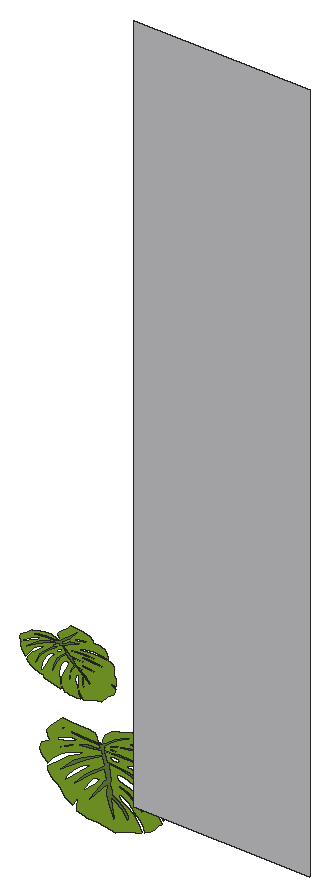
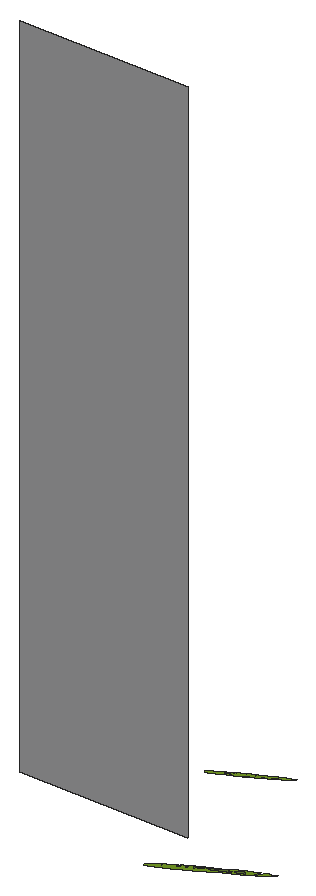
# SketchUp Ruby script. Lengths in inches.
U = 1.inch
M = Sketchup.active_model
def pt(a) = Geom::Point3d.new(a.map { |v| v * U })
def face(e, loops, mat)
  f = e.add_face(loops[0].map { |a| pt(a) })
  loops[1..].each { |l| e.add_face(l.map { |a| pt(a) }).erase! }
  f.material = f.back_material = mat if mat
  f
end
# faces: each face lists its corners as indices into pts; further lists are holes
def faces(e, pts, list, mat = nil) = list.each { |f| face(e, (f[0].is_a?(Array) ? f : [f]).map { |l| l.map { |i| pts[i] } }, mat) }
# xy, xz, yz: faces in a plane at the given z, y or x. An outline is a flat list of corners, or four numbers for a rectangle; further outlines are holes
def ring(l) = l.size == 4 ? [[l[0], l[1]], [l[2], l[1]], [l[2], l[3]], [l[0], l[3]]] : l.each_slice(2).to_a
def flat(e, list, mat, &to3) = list.each { |f| face(e, (f[0].is_a?(Array) ? f : [f]).map { |l| ring(l).map { |u, v| to3.(u, v) } }, mat) }
def xy(e, z, list, mat = nil) = flat(e, list, mat) { |x, y| [x, y, z] }
def xz(e, y, list, mat = nil) = flat(e, list, mat) { |x, z| [x, y, z] }
def yz(e, x, list, mat = nil) = flat(e, list, mat) { |y, z| [x, y, z] }
def lines(e, pts, list) = list.each { |a, b| e.add_line(pt(pts[a]), pt(pts[b])) }
# prism: a flat outline (further loops are holes) pulled along v
def prism(e, loops, v, mat = nil)
  f = face(e, loops, mat); d = Geom::Vector3d.new(v.map { |x| x * U })
  f.pushpull(f.normal.samedirection?(d) ? d.length : -d.length)
end
def box(e, o, s, mat = nil) = prism(e, [[o, [o[0] + s[0], o[1], o[2]], [o[0] + s[0], o[1] + s[1], o[2]], [o[0], o[1] + s[1], o[2]]]], [0, 0, s[2]], mat)
def at(x, y, z, deg = 0) = Geom::Transformation.translation(pt([x, y, z])) * Geom::Transformation.rotation(ORIGIN, Z_AXIS, deg.degrees)
def axes(o, x, y, z) = Geom::Transformation.new([*x, 0, *y, 0, *z, 0, *pt(o).to_a, 1])
def part(name) = M.definitions.add(name)
# library, detail: a bought-in or finely detailed component or shape, given as its bounding box
def library(name, o, s) = part(name).tap { |d| box(d.entities, o, s) }
def detail(e, o, s) = box(e.add_group.entities, o, s)
def put(e, d, t, mat = nil) = e.add_instance(d, t).tap { |i| i.material = mat if mat }
def group(e, t, mat = nil) = e.add_group.tap { |g| g.transformation = t; g.material = mat if mat }.entities
root = M.entities
M.materials.add("[0059_DarkOliveGreen]").color = [85, 107, 47]
M.materials.add("[0061_OliveDrab]").color = [107, 142, 35]
M.materials.add("[Polished Concrete New]").color = [200, 200, 203]
xz(root,148.8,[[547.38,7.8125,584.28,155.375]],"[Polished Concrete New]")
p = [[526.03,158.54,12.29],[524.84,158.39,12.53],[524.12,156.41,11.83],[524.16,155.22,11.28],[524.77,154.53,10.82],[525.48,154.2,10.48],
  [524.78,153.11,10.18],[525.2,152.12,9.62],[525.96,151.55,9.17],[527.39,151.0625,8.58],[527.87,150.84,8.36],[527.96,152.03,8.87],
  [528.62,153.25,9.25],[529.63,154.43,9.52],[530.89,155.28,9.58],[531.28,155.4375,9.55],[531.42,155.37,9.48],[531.26,155.08,9.39],
  [529.98,153.69,9.1],[529.14,152.47,8.77],[528.45,151.15,8.35],[528.24,150.44,8.09],[528.55,149.84,7.74],[529.26,149.51,7.41],
  [530.45,149.15,6.94],[531.53,148.86,6.53],[532.09,148.71,6.32],[533.02,148.16,5.83],[534.1,147.77,5.38],[535.19,147.54,5],
  [535.77,147.39,4.78],[535.6875,148.05,5.1],[535.58,149.06,5.58],[536.6875,147.26,4.49],[537,147.05,4.3125],[538.01,146.99,4.02],
  [539.03,146.92,3.73],[541.36,147.39,3.34],[544.66,147.61,2.59],[546,148.72,2.75],[547.33,149.5,2.75],[548.19,149.9375,2.73],
  [546.53,151.07,3.66],[545.23,151.69,4.28],[543.36,152.125,4.95],[542.05,152.39,5.41],[541.4,152.69,5.71],[540.88,152.94,5.96],
  [540.88,153.11,6.03],[541.24,153.17,5.97],[542.27,153.04,5.64],[543.15,152.82,5.32],[544.96,152.125,4.54],[546.48,151.5,3.87],
  [547.4375,151.15,3.46],[548.07,150.74,3.12],[548.54,150.3125,2.81],[549.22,150.98,2.93],[549.54,151.56,3.11],[549.71,152.07,3.29],
  [549.79,152.48,3.46],[549.96,152.96,3.625],[548.47,153.84,4.41],[547.06,154.3125,4.98],[545.82,154.53,5.4],[543.51,154.78,6.1],
  [541.76,154.85,6.59],[540.27,154.95,7.02],[539.16,155.1,7.37],[538.63,155.35,7.62],[538.6,155.6875,7.78],[539.43,155.83,7.625],
  [540.57,155.92,7.37],[542.57,155.75,6.78],[544.72,155.32,6.04],[547.1,154.65,5.125],[549.78,153.62,3.97],[550.08,155.34,4.67],
  [550.12,156.36,5.11],[549.7,156.81,5.42],[548.72,157.28,5.88],[547.51,157.55,6.32],[545.89,157.65,6.78],[544.51,157.73,7.17],
  [542.47,157.82,7.73],[540.96,157.76,8.1],[539.78,157.71,8.38],[539.21,157.64,8.5],[538.88,157.8,8.65],[539.23,158.04,8.67],
  [540.1,158.34,8.58],[541.47,158.49,8.29],[544.24,158.36,7.52],[545.87,158.17,7.02],[547.32,157.92,6.53],[547.99,157.67,6.25],
  [549.33,157.28,5.73],[549.38,157.5625,5.84],[549.05,158.55,6.37],[548.7,159.44,6.86],[547.35,160.44,7.66],[545.9375,160.625,8.1],
  [543.68,160.48,8.62],[541.69,160.07,8.94],[539.875,159.76,9.28],[539.08,159.61,9.41],[538.63,159.64,9.54],[538.68,159.8125,9.61],
  [539.6,160.1875,9.54],[541.83,160.71,9.2],[543.63,160.86,8.8],[546.51,160.86,8.06],[545.06,162.05,8.97],[543.6,162.67,9.62],
  [542.37,162.77,9.99],[541.74,162.57,10.06],[539.83,161.91,10.25],[538.42,161.31,10.35],[537.31,160.93,10.46],[536.86,160.88,10.55],
  [536.72,161.05,10.66],[536.96,161.21,10.68],[538.74,162.01,10.58],[540.17,162.47,10.41],[541.44,162.76,10.22],[542.41,162.97,10.0625],
  [541.22,163.4,10.5625],[540.11,163.53,10.91],[538.68,163.35,11.19],[537.34,162.96,11.36],[535.97,162.69,11.6],[535.26,162.21,11.5625],
  [534.08,161.625,11.6],[533.07,160.94,11.56],[532.59,160.04,11.28],[532.73,159.09,10.82],[533.07,158.55,10.48],[532.39,158.34,10.57],
  [531.81,158.8,10.92],[530.84,159.26,11.375],[529.57,159.23,11.6875],[527.72,158.88,12.01],[529.53,157.37,10.86],[526.06,157.09,11.63],
  [528.29,157.48,11.23],[532.95,158.28,10.39],[533.52,158.98,10.5625],[534.42,160.48,11],[535.61,161.42,11.12],[536.63,161.96,11.1],
  [535.04,160.39,10.8],[534.11,159.09,10.46],[533.82,158.37,10.21],[535.125,159.53,10.39],[537.7,160.62,10.22],[539.75,161.2,9.95],
  [541.875,161.65,9.61],[542.9375,161.78,9.39],[539.66,160.88,9.83],[537.71,160.24,10.05],[535.5625,159.37,10.21],[534.45,158.62,10.16],
  [533.99,158.19,10.09],[534.1,157.93,9.94],[534.45,157.87,9.82],[535.4,158.125,9.69],[536.36,158.53,9.63],[537.48,158.8,9.46],
  [540.75,159.32,8.85],[542.84,159.49,8.39],[544.79,159.34,7.82],[546.375,159.24,7.37],[546.97,158.95,7.09],[543.92,159.16,7.96],
  [542.19,159.1,8.38],[539.46,158.8,8.95],[537.05,158.31,9.35],[534.42,157.63,9.72],[535.79,156.5625,8.89],[537.83,156.82,8.48],
  [539.75,157.03,8.08],[543.72,156.83,6.97],[545.69,156.45,6.29],[547.01,156.125,5.81],[547.625,155.83,5.52],[545.76,156.18,6.16],
  [542.69,156.5,7.09],[538.76,156.6,8.14],[536.41,156.27,8.6],[538.51,154.23,7.14],[540.09,154.38,6.8],[542.03,154.17,6.21],
  [543.89,153.72,5.53],[545.29,153.24,4.95],[546.83,152.5,4.23],[543.64,153.54,5.51],[541.8,153.96,6.18],[540.09,154.09,6.68],
  [538.53,153.99,7.03],[539.87,152.4,5.97],[541.58,152.11,5.4],[543.1,151.61,4.79],[544.35,151.02,4.2],[544.9,150.4375,3.8],
  [542.81,151.43,4.78],[541.24,151.83,5.37],[539.98,152.0625,5.79],[541.28,150.83,4.91],[541.95,150.16,4.43],[542.93,149.32,3.8],
  [542.75,149.43,3.9],[540.875,150.67,4.94],[539.38,151.94,5.89],[538.25,153.45,6.86],[537.48,149.88,5.46],[537.49,153.95,7.28],
  [536.15,155.16,8.17],[534.93,153.42,7.7],[533.69,150.58,6.75],[534.14,152.67,7.57],[535.05,154.6,8.2],[535.79,155.61,8.46],
  [534.48,156.625,9.26],[532.34,154.42,8.82],[530.24,151.21,7.92],[531.1,153.79,8.85],[532.58,155.49,9.24],[534.21,156.9375,9.47],
  [533.77,157.36,9.77],[532.13,156.78,9.93],[529.95,156.02,10.15],[527.76,154.28,9.93],[529.26,155.84,10.25],[530.98,157,10.33],
  [532.92,157.45,10.03],[533.23,157.66,10.05],[532.59,157.97,10.34],[532.34,152.84,8.11],[533.07,154.03,8.45],[533.45,154.32,8.49],
  [533.72,154.38,8.45],[533.83,154.25,8.36],[533.61,153.77,8.2],[533.08,152.65,7.83],[532.51,151.41,7.42],[532.07,150.1,6.95],
  [531.84,149.48,6.73],[531.91,151.34,7.55],[535.73,152.99,7.3],[536.08,153.41,7.4],[536.47,153.43,7.3125],[536.6875,153.25,7.17],
  [536.72,152.83,6.98],[536.58,152.5,6.87],[536.07,151.19,6.41],[535.58,149.97,5.99],[535.51,151.84,6.84],[527.14,155.96,10.84],
  [528.12,156.47,10.83],[528.97,156.77,10.74],[529.43,156.74,10.61],[529.58,156.61,10.51],[528.15,155.72,10.48],[526.88,155.02,10.49],
  [526.51,154.88,10.53],[526.54,155.39,10.74],[536.13,157.73,9.33],[536.87,157.78,9.16],[537.42,157.62,8.95],[537.37,157.4,8.86],
  [536.67,157.16,8.93],[535.8125,157.21,9.18],[535.54,157.47,9.36],[534.86,158.61,10.05],[535.62,158.79,9.9375],[536.18,158.8,9.79],
  [536.16,158.57,9.7],[535.34,158.38,9.82],[534.73,158.36,9.97],[532.04,157.45,29.43],[533.29,157.72,29.23],[534.4375,157.5625,28.86],
  [535.09,157.27,28.57],[535.65,156.73,28.18],[535.91,156.55,28.03],[534.54,156.51,28.37],[533.13,156.27,28.62],[531.78,155.88,28.79],
  [530.8,155.41,28.83],[530.62,155.26,28.8125],[530.69,155.21,28.77],[531.03,155.27,28.71],[532.62,155.75,28.52],[534.03,156.07,28.3],
  [535.55,156.33,28.02],[536.36,156.41,27.85],[537.06,156.29,27.62],[537.44,156.02,27.4],[537.85,155.57,27.09],[538.1875,155.16,26.82],
  [538.36,154.95,26.68],[538.99,154.6,26.36],[539.43,154.19,26.0625],[539.7,153.78,25.81],[539.88,153.56,25.67],[539.11,153.59,25.875],
  [537.96,153.63,26.19],[540.02,153.21,25.47],[540.27,153.09,25.36],[540.34,152.71,25.17],[540.41,152.33,24.97],[539.88,151.44,24.72],
  [539.62,150.19,24.22],[538.34,149.6875,24.32],[537.45,149.18,24.33],[536.95,148.86,24.31],[535.64,149.49,24.93],[534.93,149.98,25.33],
  [534.43,150.68,25.78],[534.125,151.18,26.08],[533.77,151.43,26.28],[533.49,151.625,26.44],[533.29,151.625,26.49],[533.23,151.49,26.45],
  [533.38,151.1,26.23],[533.63,150.77,26.02],[534.43,150.08,25.51],[535.15,149.51,25.0625],[535.55,149.14,24.8],[536.02,148.9,24.57],
  [536.51,148.73,24.36],[535.74,148.47,24.45],[535.08,148.35,24.5625],[534.49,148.28,24.68],[534.02,148.25,24.79],[533.47,148.1875,24.9],
  [532.45,148.75,25.42],[531.91,149.29,25.8],[531.66,149.75,26.07],[531.375,150.63,26.54],[531.29,151.29,26.86],[531.17,151.86,27.14],
  [531.01,152.28,27.37],[530.72,152.48,27.54],[530.33,152.49,27.64],[530.16,152.17,27.54],[530.06,151.74,27.375],[530.25,150.98,26.99],
  [530.75,150.17,26.5],[531.52,149.27,25.89],[532.71,148.26,25.13],[530.73,148.14,25.59],[529.55,148.125,25.89],[529.04,148.29,26.09],
  [528.5,148.66,26.39],[528.19,149.11,26.68],[528.07,149.73,26.99],[527.98,150.25,27.24],[527.88,151.02,27.62],[527.95,151.59,27.85],
  [528,152.04,28.04],[528.08,152.26,28.12],[527.9,152.38,28.22],[527.62,152.25,28.23],[527.28,151.92,28.17],[527.11,151.4,27.98],
  [527.25,150.35,27.48],[527.47,149.74,27.14],[527.76,149.19,26.82],[528.04,148.93,26.64],[528.5,148.43,26.29],[528.17,148.41,26.37],
  [527.03,148.53,26.72],[526.02,148.66,27.04],[524.86,149.17,27.5625],[524.65,149.71,27.86],[524.81,150.57,28.2],[525.29,151.32,28.41],
  [525.64,152,28.63],[525.82,152.31,28.72],[525.78,152.48,28.81],[525.58,152.46,28.85],[525.15,152.11,28.81],[524.55,151.27,28.58],
  [524.37,150.58,28.32],[524.38,149.49,27.83],[523.01,150.04,28.43],[522.29,150.6,28.86],[522.17,151.0625,29.1],[522.4,151.3,29.15],
  [523.16,152.02,29.28],[523.86,152.56,29.34],[524.3,152.98,29.41],[524.35,153.15,29.48],[524.16,153.2,29.55],[523.97,153.11,29.56],
  [523.05,152.44,29.49],[522.53,151.89,29.38],[522.18,151.41,29.26],[521.95,151.05,29.15],[521.45,151.5,29.48],[521.3,151.91,29.71],
  [521.51,152.46,29.9],[521.96,152.96,30.01],[522.26,153.48,30.16],[522.82,153.75,30.14],[523.49,154.2,30.17],[524.28,154.58,30.14],
  [525.32,154.76,29.95],[526.41,154.71,29.65],[527.04,154.58,29.43],[527.27,154.84,29.48],[526.75,155.06,29.72],[526.22,155.43,30.02],
  [526.25,155.91,30.23],[526.65,156.6,30.4375],[527.05,157.24,30.62],[527.22,157.7,30.78],[529.49,157.97,30.32],[530.86,157.95,29.96],
  [531.66,157.72,29.65],[535.48,155.65,27.74],[532.52,155.33,28.35],[530.56,154.77,28.61],[528.89,154.15,28.76],[528.41,154.3125,28.96],
  [529.07,154.93,29.0625],[529.95,155.76,29.21],[531.95,156.59,29.07],[530.15,156.02,29.27],[528.82,155.375,29.33],[528.3,154.64,29.13],
  [528.05,154.52,29.14],[527.7,154.76,29.34],[528.4,155.92,29.68],[528.71,157.23,30.19],[527.34,154.625,29.37],[526.54,154.41,29.48],
  [524.8125,154.07,29.77],[523.73,153.62,29.85],[523.11,153.23,29.84],[524.92,153.84,29.64],[526.41,154.1875,29.41],[527.25,154.3,29.25],
  [525.91,153.8,29.37],[524.65,152.83,29.26],[523.99,152.05,29.08],[523.47,151.25,28.85],[523.3125,150.85,28.71],[524.35,152.09,29],
  [525.09,152.82,29.14],[526.09,153.64,29.25],[526.96,154.06,29.22],[527.45,154.23,29.17],[527.75,154.19,29.07],[527.82,154.06,28.99],
  [527.52,153.7,28.91],[527.05,153.34,28.87],[526.74,152.91,28.76],[526.14,151.67,28.35],[525.95,150.88,28.05],[526.13,150.14,27.67],
  [526.24,149.54,27.375],[526.57,149.32,27.1875],[526.33,150.47,27.77],[526.41,151.13,28.04],[526.75,152.16,28.42],[527.3125,153.07,28.68],
  [528.09,154.07,28.93],[529.32,153.55,28.38],[529.02,152.78,28.11],[528.78,152.05,27.85],[529.02,150.55,27.11],[529.45,149.8,26.66],
  [529.82,149.3,26.34],[530.16,149.07,26.15],[529.76,149.78,26.57],[529.4,150.9375,27.1875],[529.28,152.43,27.88],[529.66,153.32,28.1875],
  [532.01,152.52,27.23],[531.83,151.92,27],[532.07,151.19,26.61],[532.59,150.49,26.16],[533.15,149.95,25.78],[533.99,149.375,25.3],
  [532.8,150.58,26.15],[532.32,151.28,26.59],[532.16,151.93,26.92],[532.28,152.51,27.15],[534.12,152.01,26.45],[534.45,151.36,26.08],
  [535.02,150.78,25.67],[535.7,150.3125,25.28],[536.37,150.1,25.02],[535.22,150.89,25.67],[534.77,151.49,26.05],[534.5,151.97,26.33],
  [535.92,151.47,25.75],[536.6875,151.22,25.4375],[537.66,150.85,25.02],[537.53,150.92,25.08],[536.1,151.625,25.77],[534.64,152.19,26.4],
  [532.9,152.62,27.04],[537.01,152.91,26.11],[532.33,152.91,27.32],[530.93,153.42,27.9],[532.94,153.875,27.59],[536.2,154.35,26.96],
  [533.8,154.18,27.51],[531.59,153.83,27.92],[530.42,153.55,28.1],[529.25,154.05,28.62],[531.78,154.86,28.33],[533.6,154.86,27.86],
  [532.24,154.58,28.09],[531.91,154.4375,28.11],[531.83,154.33,28.08],[531.99,154.29,28.03],[532.53,154.375,27.92],[533.83,154.58,27.68],
  [535.26,154.79,27.41],[536.76,154.96,27.1],[537.47,155.05,26.95],[535.33,155.02,27.49],[533.4375,153.57,27.33],[532.95,153.44,27.4],
  [532.92,153.29,27.34],[533.13,153.21,27.25],[533.62,153.2,27.12],[533.99,153.25,27.04],[535.5,153.45,26.74],[536.9,153.63,26.46],
  [534.76,153.66,27.03],[530.67,157.05,29.6],[530.02,156.82,29.67],[529.42,156.46,29.66],[529.08,156.13,29.6],[529.11,155.96,29.51],
  [529.27,155.9,29.45],[530.29,156.44,29.43],[531.1,156.92,29.43],[531.25,157.0625,29.46],[528.36,152.95,28.36],[528.64,153.22,28.41],
  [528.57,153.54,28.57],[528.27,153.64,28.69],[527.98,153.42,28.67],[527.92,153.14,28.56],[528.1,152.93,28.42],[526.97,153.9,29.14],
  [526.76,153.62,29.07],[526.75,153.4,28.97],[527.01,153.41,28.91],[527.23,153.72,28.99],[527.25,153.95,29.09]]
faces(root,p,[[[0,1,2,3,4,5,6,7,8,9,10,11,12,13,14,15,16,17,18,19,20,21,22,23,24,25,26,27,28,29,30,31,32,33,34,35,36,37,38,39,40,41,42,43,44,45,46,47,48,49,50,51,52,53,54,55,56,57,58,59,60,61,62,63,64,65,66,67,68,69,70,71,72,73,74,75,76,77,78,79,80,81,82,83,84,85,86,87,88,89,90,91,92,93,94,95,80,96,97,98,99,100,101,102,103,104,105,106,107,108,109,110,111,112,113,114,115,116,117,118,119,120,121,122,123,124,125,126,127,128,129,130,131,132,133,134,135,136,137,138,139,140,141],[142,143,144,145,146,147,148,149,150,151,152,153,154,155,156,157,158,159,160,161,162,163,164,165,166,167,168,169,170,171,172,173,174,175,176,177,178,179,180,181,182,183,184,185,186,187,188,189,190,191,192,193,194,195,196,197,198,199,200,201,202,203,204,205,206,207,208,209,210,211,212,213,214,215,216,217,218,219,220,221,222,223,224,225,226,227,228,229,230,231,232,233,234,235,236],[237,238,239,240,241,242,243,244,245,246,247],[248,249,250,251,252,253,254,255,256],[257,258,259,260,261,262,263,264,265],[266,267,268,269,270,271,272],[273,274,275,276,277,278]],[[279,280,281,282,283,284,285,286,287,288,289,290,291,292,293,294,295,296,297,298,299,300,301,302,303,304,305,306,307,308,309,310,311,312,313,314,315,316,317,318,319,320,321,322,323,324,325,326,327,328,329,330,331,332,333,334,335,336,337,338,339,340,341,342,343,344,345,346,347,348,349,350,351,352,353,354,355,356,357,358,359,360,361,362,363,364,365,366,367,368,369,354,370,371,372,373,374,375,376,377,378,379,380,381,382,383,384,385,386,387,388,389,390,391,392,393,394,395,396,397,398,399,400,401,402,403,404,405,406,407,408,409,410,411,412,413,414,415,416,417,418,419,420],[421,422,423,424,425,426,427,428,429,430,431,432,433,434,435,436,437,438,439,440,441,442,443,444,445,446,447,448,449,450,451,452,453,454,455,456,457,458,459,460,461,462,463,464,465,466,467,468,469,470,471,472,473,474,475,476,477,478,479,480,481,482,483,484,485,486,487,488,489,490,491,492,493,494,495,496,497,498,499,500,501,502,503,504,505,506,507,508,509,510,511,512,513,514],[515,516,517,518,519,520,521,522,523,524,525],[526,527,528,529,530,531,532,533,534],[535,536,537,538,539,540,541,542,543],[544,545,546,547,548,549,550],[551,552,553,554,555,556]]],"[0061_OliveDrab]")
faces(root,p,[[143,142,236,235,234,233,232,231,230,229,228,227,226,225,224,223,222,221,220,219,218,217,216,215,214,213,212,211,210,209,208,207,206,205,204,203,202,201,200,199,198,197,196,195,194,193,192,191,190,189,188,187,186,185,184,183,182,181,180,179,178,177,176,175,174,173,172,171,170,169,168,167,166,165,164,163,162,161,160,159,158,157,156,155,154,153,152,151,150,149,148,147,146,145,144],[422,421,514,513,512,511,510,509,508,507,506,505,504,503,502,501,500,499,498,497,496,495,494,493,492,491,490,489,488,487,486,485,484,483,482,481,480,479,478,477,476,475,474,473,472,471,470,469,468,467,466,465,464,463,462,461,460,459,458,457,456,455,454,453,452,451,450,449,448,447,446,445,444,443,442,441,440,439,438,437,436,435,434,433,432,431,430,429,428,427,426,425,424,423]],"[0059_DarkOliveGreen]")
